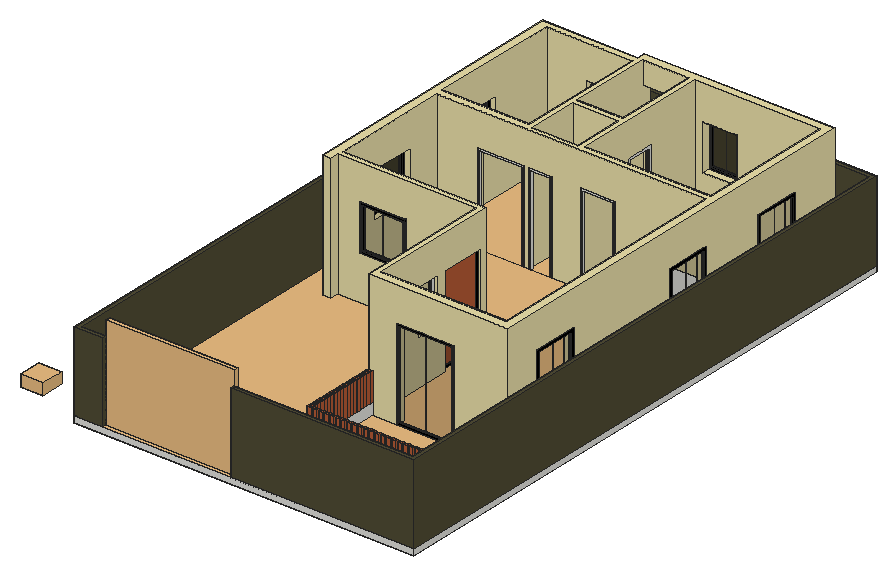
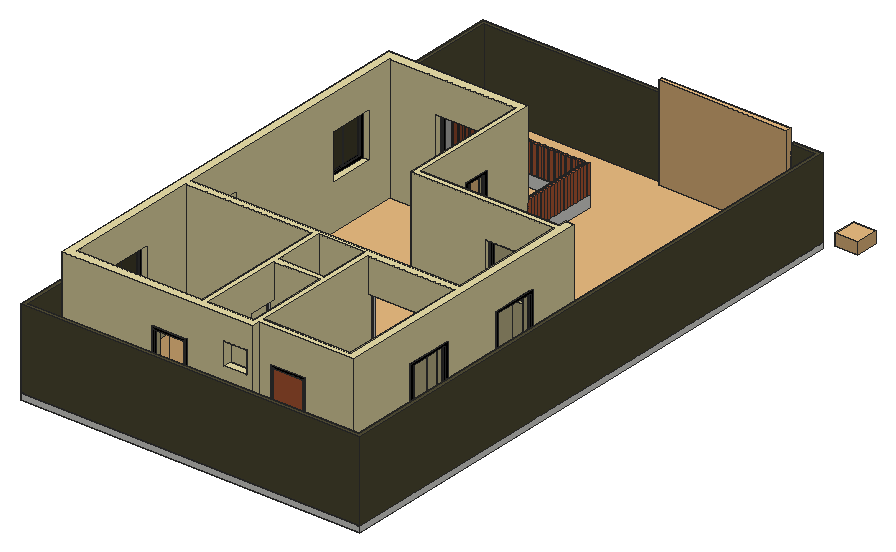
# SketchUp Ruby script. Lengths in inches.
U = 1.inch
M = Sketchup.active_model
def pt(a) = Geom::Point3d.new(a.map { |v| v * U })
def face(e, loops, mat)
  f = e.add_face(loops[0].map { |a| pt(a) })
  loops[1..].each { |l| e.add_face(l.map { |a| pt(a) }).erase! }
  f.material = f.back_material = mat if mat
  f
end
# faces: each face lists its corners as indices into pts; further lists are holes
def faces(e, pts, list, mat = nil) = list.each { |f| face(e, (f[0].is_a?(Array) ? f : [f]).map { |l| l.map { |i| pts[i] } }, mat) }
# xy, xz, yz: faces in a plane at the given z, y or x. An outline is a flat list of corners, or four numbers for a rectangle; further outlines are holes
def ring(l) = l.size == 4 ? [[l[0], l[1]], [l[2], l[1]], [l[2], l[3]], [l[0], l[3]]] : l.each_slice(2).to_a
def flat(e, list, mat, &to3) = list.each { |f| face(e, (f[0].is_a?(Array) ? f : [f]).map { |l| ring(l).map { |u, v| to3.(u, v) } }, mat) }
def xy(e, z, list, mat = nil) = flat(e, list, mat) { |x, y| [x, y, z] }
def xz(e, y, list, mat = nil) = flat(e, list, mat) { |x, z| [x, y, z] }
def yz(e, x, list, mat = nil) = flat(e, list, mat) { |y, z| [x, y, z] }
def lines(e, pts, list) = list.each { |a, b| e.add_line(pt(pts[a]), pt(pts[b])) }
# prism: a flat outline (further loops are holes) pulled along v
def prism(e, loops, v, mat = nil)
  f = face(e, loops, mat); d = Geom::Vector3d.new(v.map { |x| x * U })
  f.pushpull(f.normal.samedirection?(d) ? d.length : -d.length)
end
def box(e, o, s, mat = nil) = prism(e, [[o, [o[0] + s[0], o[1], o[2]], [o[0] + s[0], o[1] + s[1], o[2]], [o[0], o[1] + s[1], o[2]]]], [0, 0, s[2]], mat)
def at(x, y, z, deg = 0) = Geom::Transformation.translation(pt([x, y, z])) * Geom::Transformation.rotation(ORIGIN, Z_AXIS, deg.degrees)
def axes(o, x, y, z) = Geom::Transformation.new([*x, 0, *y, 0, *z, 0, *pt(o).to_a, 1])
def part(name) = M.definitions.add(name)
# library, detail: a bought-in or finely detailed component or shape, given as its bounding box
def library(name, o, s) = part(name).tap { |d| box(d.entities, o, s) }
def detail(e, o, s) = box(e.add_group.entities, o, s)
def put(e, d, t, mat = nil) = e.add_instance(d, t).tap { |i| i.material = mat if mat }
def group(e, t, mat = nil) = e.add_group.tap { |g| g.transformation = t; g.material = mat if mat }.entities
root = M.entities
M.materials.add("METAL").color = [0, 0, 0]
M.materials.add("WALL PAINT").color = [235, 224, 170]
M.materials.add("WALL PAINT\#1").color = [80, 76, 53]
M.materials.add("WHITE FLOOR").color = [250, 250, 243]
M.materials.add("glass").color = [0, 0, 0]
M.materials["glass"].alpha = 0.1
M.materials.add("wood").color = [181, 91, 54]
c1 = part("Group\#111")
box(c1.entities,[0,0,0],[4.5,2.78,30])
c2 = part("Stair tread")
box(c2.entities,[0,0,0],[12,39.4375,7])
c3 = library("gate 119k",[0,1.18,0],[135.43,4.73,99.21])
c4 = library("Group\#1",[0,0,0],[357,609,0.01])
c5 = library("Dome Light",[-12,-12,0],[24,24,12])
c6 = part("Component\#2")
box(c6.entities,[0,0,0],[36,36,19.4375])
prism(root,[[[164.87,4.5,0],[352.5,4.5,0],[352.5,604.5,0],[4.5,604.5,0],[4.5,4.5,0],[29.875,4.5,0],[29.875,0,0],[0,0,0],[0,609,0],[357,609,0],[357,0,0],[164.87,0,0]]],[0,0,84],"WALL PAINT\#1")
g1 = group(root,at(32,74,-6))
xy(g1,0,[[-32,-74,325,535]])
xy(g1,6,[[-32,-74,325,535]],"WHITE FLOOR")
xz(g1,-74,[[-32,0,325,6]])
xz(g1,535,[[-32,0,325,6]])
yz(g1,-32,[[-74,0,535,6]])
yz(g1,325,[[-74,0,535,6]])
g2 = group(root,at(216,154.5,0))
prism(g2,[[[60,0,95.4375],[0,0,95.4375],[0,0,0],[60,0,0]],[[58,0,2],[2,0,2],[2,0,93.4375],[58,0,93.4375]]],[0,2,0],"METAL")
g3 = group(root,at(138,426,0))
prism(g3,[[[2,2,0],[0,2,0],[0,2,95.4375],[24,2,95.4375],[24,2,0],[22,2,0],[22,2,93.4375],[2,2,93.4375]]],[0,-2,0])
p = [[2,0,0],[22,0,0]]
lines(g3,p,[[0,1]])
g4 = group(root,at(192,426,0))
prism(g4,[[[2,2,0],[0,2,0],[0,2,95.4375],[36,2,95.4375],[36,2,0],[34,2,0],[34,2,93.4375],[2,2,93.4375]]],[0,-2,0])
p = [[2,0,0],[34,0,0]]
lines(g4,p,[[0,1]])
g5 = group(root,at(186,74,0))
xy(g5,0,[[0,0,0,80.5,4.5,80.5,4.5,4.5,142.5,4.5,142.5,80.5,147,80.5,147,0]])
xy(g5,12,[[0,0,147,0,147,4.5,4.5,4.5,4.5,77.72,0,77.72]])
xy(g5,48,[[142.5,4.5,147,80.5]])
xz(g5,0,[[0,0,147,12]])
xz(g5,4.5,[[4.5,0,142.5,12],[142.5,12,147,48]])
xz(g5,80.5,[[0,0,4.5,12],[142.5,0,147,48]])
yz(g5,0,[[0,0,80.5,12]])
yz(g5,4.5,[[4.5,0,80.5,12]])
yz(g5,142.5,[[4.5,0,80.5,48]])
yz(g5,147,[[0,0,80.5,0,80.5,48,4.5,48,4.5,12,0,12]])
put(g5,c1,at(0,77.72,12),"wood")
put(g5,c1,at(0,73.4,12),"wood")
put(g5,c1,at(0,69.08,12),"wood")
g6 = group(g5,at(0,64.77,12),"wood")
box(g6,[0,0,0],[4.5,2.78,30])
put(g5,c1,at(0,60.45,12),"wood")
put(g5,c1,at(0,56.13,12),"wood")
put(g5,c1,at(0,51.8125,12),"wood")
put(g5,c1,at(0,47.49,12),"wood")
put(g5,c1,at(0,43.18,12),"wood")
put(g5,c1,at(0,38.86,12),"wood")
put(g5,c1,at(0,34.54,12),"wood")
put(g5,c1,at(0,30.22,12),"wood")
put(g5,c1,at(0,25.91,12),"wood")
put(g5,c1,at(0,21.59,12),"wood")
put(g5,c1,at(0,17.27,12),"wood")
put(g5,c1,at(0,12.95,12),"wood")
put(g5,c1,at(0,8.64,12),"wood")
put(g5,c1,at(0,4.32,12),"wood")
put(g5,c1,at(0,0,12),"wood")
put(g5,c1,at(5.9375,0,12),"wood")
put(g5,c1,at(11.875,0,12),"wood")
put(g5,c1,at(17.8125,0,12),"wood")
put(g5,c1,at(23.75,0,12),"wood")
put(g5,c1,at(29.6875,0,12),"wood")
put(g5,c1,at(35.625,0,12),"wood")
put(g5,c1,at(41.5625,0,12),"wood")
put(g5,c1,at(47.5,0,12),"wood")
put(g5,c1,at(53.4375,0,12),"wood")
put(g5,c1,at(59.375,0,12),"wood")
put(g5,c1,at(65.3125,0,12),"wood")
put(g5,c1,at(71.25,0,12),"wood")
put(g5,c1,at(77.1875,0,12),"wood")
put(g5,c1,at(83.125,0,12),"wood")
put(g5,c1,at(89.0625,0,12),"wood")
put(g5,c1,at(95,0,12),"wood")
put(g5,c1,at(100.9375,0,12),"wood")
put(g5,c1,at(106.875,0,12),"wood")
put(g5,c1,at(112.8125,0,12),"wood")
put(g5,c1,at(118.75,0,12),"wood")
put(g5,c1,at(124.6875,0,12),"wood")
put(g5,c1,at(130.625,0,12),"wood")
put(g5,c1,at(136.5625,0,12),"wood")
put(g5,c1,at(142.5,0,12),"wood")
put(root,c2,at(228,390,0))
put(root,c3,at(29.875,3.32,0))
g7 = group(root,at(32,154.5,0))
xy(g7,0,[[244,0,244,9,292,9,292,271.5,196,271.5,196,277.5,292,277.5,292,421.5,160,421.5,160,364.5,154,364.5,154,421.5,106,421.5,106,271.5,100,271.5,100,430.5,301,430.5,301,0],[154,0,154,92.9375,160,92.9375,160,9,184,9,184,0],[0,132,0,421.5,52,421.5,52,415.5,9,415.5,9,278.5,52,278.5,52,271.5,9,271.5,9,147,160,147,160,141,9,141,9,132]],"WALL PAINT")
xy(g7,47.4375,[[292,36.07,301,84.07],[154,57,160,83.9375],[33,141,81,147],[0,188.67,9,236.67],[292,210.97,301,258.97],
  [0,301.21,9,349.21],[292,327.45,301,375.45],[169,421.5,205,430.5]],"WALL PAINT")
xy(g7,83.4375,[[106,421.5,130,430.5]],"WALL PAINT")
xy(g7,95.4375,[[184,0,244,9],[292,36.07,301,84.07],[154,57,160,83.9375],[154,92.9375,160,141],[33,141,81,147],
  [0,188.67,9,236.67],[292,210.97,301,258.97],[52,271.5,100,278.5],[106,271.5,130,275.5],[160,271.5,196,277.5],
  [0,301.21,9,349.21],[292,327.45,301,375.45],[154,334.5,160,364.5],[52,415.5,88,421.5],[169,421.5,205,430.5]],"WALL PAINT")
xy(g7,107.4375,[[106,421.5,130,430.5]],"WALL PAINT")
xy(g7,131.4375,[[[154,0,301,0,301,430.5,100,430.5,100,421.5,0,421.5,0,132,9,132,9,141,154,141],[160,9,160,147,9,147,9,271.5,292,271.5,292,9],[160,277.5,292,421.5],[9,278.5,100,415.5],[106,334.5,154,421.5],[106,275.5,154,328.5]]],"WALL PAINT")
xz(g7,0,[[154,0,184,0,184,95.4375,244,95.4375,244,0,301,0,301,131.4375,154,131.4375]],"WALL PAINT")
xz(g7,9,[[160,0,160,131.4375,292,131.4375,292,0,244,0,244,95.4375,184,95.4375,184,0]],"WALL PAINT")
xz(g7,36.07,[[292,47.4375,301,95.4375]],"WALL PAINT")
xz(g7,57,[[154,47.4375,160,95.4375]],"WALL PAINT")
xz(g7,83.9375,[[154,47.4375,160,95.4375]],"WALL PAINT")
xz(g7,84.07,[[292,47.4375,301,95.4375]],"WALL PAINT")
xz(g7,92.9375,[[154,0,160,95.4375]],"WALL PAINT")
xz(g7,132,[[0,0,9,131.4375]],"WALL PAINT")
xz(g7,141,[[[9,0,160,0,160,95.4375,154,95.4375,154,131.4375,9,131.4375],[33,47.4375,81,95.4375]]],"WALL PAINT")
xz(g7,147,[[[9,0,160,131.4375],[33,47.4375,81,95.4375]]],"WALL PAINT")
xz(g7,188.67,[[0,47.4375,9,95.4375]],"WALL PAINT")
xz(g7,210.97,[[292,47.4375,301,95.4375]],"WALL PAINT")
xz(g7,236.67,[[0,47.4375,9,95.4375]],"WALL PAINT")
xz(g7,258.97,[[292,47.4375,301,95.4375]],"WALL PAINT")
xz(g7,271.5,[[9,0,52,0,52,95.4375,100,95.4375,100,0,106,0,106,95.4375,130,95.4375,130,0,160,0,160,95.4375,196,95.4375,196,0,292,0,292,131.4375,9,131.4375]],"WALL PAINT")
xz(g7,275.5,[[130,0,130,95.4375,106,95.4375,106,131.4375,154,131.4375,154,0]],"WALL PAINT")
xz(g7,277.5,[[196,0,196,95.4375,160,95.4375,160,131.4375,292,131.4375,292,0]],"WALL PAINT")
xz(g7,278.5,[[9,0,9,131.4375,100,131.4375,100,95.4375,52,95.4375,52,0]],"WALL PAINT")
xz(g7,301.21,[[0,47.4375,9,95.4375]],"WALL PAINT")
xz(g7,327.45,[[292,47.4375,301,95.4375]],"WALL PAINT")
xz(g7,328.5,[[106,0,154,131.4375]],"WALL PAINT")
xz(g7,334.5,[[106,0,106,131.4375,154,131.4375,154,95.4375,160,95.4375,160,0]],"WALL PAINT")
xz(g7,349.21,[[0,47.4375,9,95.4375]],"WALL PAINT")
xz(g7,364.5,[[154,0,160,95.4375]],"WALL PAINT")
xz(g7,375.45,[[292,47.4375,301,95.4375]],"WALL PAINT")
xz(g7,415.5,[[9,0,52,0,52,95.4375,88,95.4375,88,0,100,0,100,131.4375,9,131.4375]],"WALL PAINT")
xz(g7,421.5,[[0,0,0,131.4375,100,131.4375,100,0,88,0,88,95.4375,52,95.4375,52,0],[106,0,154,0,154,131.4375,106,131.4375,106,107.4375,130,107.4375,130,83.4375,106,83.4375],[[160,0,292,131.4375],[169,47.4375,205,95.4375]]],"WALL PAINT")
xz(g7,430.5,[[[100,0,301,131.4375],[169,47.4375,205,95.4375],[106,83.4375,130,107.4375]]],"WALL PAINT")
yz(g7,0,[[[132,0,421.5,131.4375],[301.21,47.4375,349.21,95.4375],[188.67,47.4375,236.67,95.4375]]],"WALL PAINT")
yz(g7,9,[[132,0,141,131.4375],[[147,0,271.5,131.4375],[188.67,47.4375,236.67,95.4375]],[[278.5,0,415.5,131.4375],[301.21,47.4375,349.21,95.4375]]],"WALL PAINT")
yz(g7,33,[[141,47.4375,147,95.4375]],"WALL PAINT")
yz(g7,52,[[271.5,0,278.5,95.4375],[415.5,0,421.5,95.4375]],"WALL PAINT")
yz(g7,81,[[141,47.4375,147,95.4375]],"WALL PAINT")
yz(g7,88,[[415.5,0,421.5,95.4375]],"WALL PAINT")
yz(g7,100,[[271.5,0,271.5,95.4375,278.5,95.4375,278.5,131.4375,415.5,131.4375,415.5,0],[421.5,0,430.5,131.4375]],"WALL PAINT")
yz(g7,106,[[271.5,0,328.5,0,328.5,131.4375,275.5,131.4375,275.5,95.4375,271.5,95.4375],[334.5,0,421.5,0,421.5,83.4375,430.5,83.4375,430.5,107.4375,421.5,107.4375,421.5,131.4375,334.5,131.4375]],"WALL PAINT")
yz(g7,130,[[271.5,0,275.5,95.4375],[421.5,83.4375,430.5,107.4375]],"WALL PAINT")
yz(g7,154,[[[0,0,0,131.4375,141,131.4375,141,95.4375,92.9375,95.4375,92.9375,0],[57,47.4375,83.9375,95.4375]],[275.5,0,328.5,131.4375],[364.5,0,364.5,95.4375,334.5,95.4375,334.5,131.4375,421.5,131.4375,421.5,0]],"WALL PAINT")
yz(g7,160,[[[9,0,92.9375,0,92.9375,95.4375,141,95.4375,141,0,147,0,147,131.4375,9,131.4375],[57,47.4375,83.9375,95.4375]],[271.5,0,334.5,0,334.5,95.4375,364.5,95.4375,364.5,0,421.5,0,421.5,131.4375,277.5,131.4375,277.5,95.4375,271.5,95.4375]],"WALL PAINT")
yz(g7,169,[[421.5,47.4375,430.5,95.4375]],"WALL PAINT")
yz(g7,184,[[0,0,9,95.4375]],"WALL PAINT")
yz(g7,196,[[271.5,0,277.5,95.4375]],"WALL PAINT")
yz(g7,205,[[421.5,47.4375,430.5,95.4375]],"WALL PAINT")
yz(g7,244,[[0,0,9,95.4375]],"WALL PAINT")
yz(g7,292,[[[9,0,271.5,131.4375],[36.07,47.4375,84.07,95.4375],[210.97,47.4375,258.97,95.4375]],[[277.5,0,421.5,131.4375],[327.45,47.4375,375.45,95.4375]]],"WALL PAINT")
yz(g7,301,[[[0,0,430.5,131.4375],[36.07,47.4375,84.07,95.4375],[210.97,47.4375,258.97,95.4375],[327.45,47.4375,375.45,95.4375]]],"WALL PAINT")
p = [[244,0,0],[184,0,0]]
lines(g7,p,[[0,1]])
put(root,c4,at(0,0,0))
g8 = group(root,at(84,576,0))
xy(g8,0,[[0,-2,36,0]])
xy(g8,2,[[2,-2,34,0]])
xy(g8,93.4375,[[2,-2,34,0]])
xy(g8,95.4375,[[0,-2,36,0]])
xz(g8,-2,[[[0,0,36,95.4375],[2,2,34,93.4375]]])
xz(g8,0,[[[0,0,36,95.4375],[2,2,34,93.4375]]],"METAL")
yz(g8,0,[[-2,0,0,95.4375]])
yz(g8,2,[[-2,2,0,93.4375]])
yz(g8,34,[[-2,2,0,93.4375]])
yz(g8,36,[[-2,0,0,95.4375]])
g9 = group(root,at(186,247.4375,0))
prism(g9,[[[0,48.0625,95.4375],[0,48.0625,0],[0,0,0],[0,0,95.4375]],[[0,46.0625,93.4375],[0,2,93.4375],[0,2,2],[0,46.0625,2]]],[2,0,0],"METAL")
g10 = group(root,at(84,426,0))
prism(g10,[[[0,0,0],[2,0,0],[2,0,93.4375],[46,0,93.4375],[46,0,0],[48,0,0],[48,0,95.4375],[0,0,95.4375]]],[0,2,0])
p = [[2,0,0],[46,0,0]]
lines(g10,p,[[0,1]])
g11 = group(root,at(192,489,0))
prism(g11,[[[0,0,0],[0,30,0],[0,30,95.4375],[0,0,95.4375]],[[0,28,93.4375],[0,28,2],[0,2,2],[0,2,93.4375]]],[-2,0,0])
g12 = group(root,at(218,155.875,2))
box(g12,[0,0,0],[28,0.31,91.4375],"glass")
g13 = group(root,at(246,155.56,2))
box(g13,[0,0,0],[28,0.31,91.4375],"glass")
g14 = group(root,at(186,249.4375,2),"wood")
box(g14,[0,0,0],[0.71,44.0625,91.4375])
g15 = group(root,at(86,576,2),"wood")
box(g15,[0,-0.71,0],[32,0.71,91.4375])
put(root,c2,at(240,390,7))
put(root,c5,at(-38.72,4.5,13.38))
put(root,c2,at(252,390,14))
put(root,c2,at(264,390,21))
put(root,c2,at(276,390,28))
put(root,c6,at(288,390,35))
g16 = group(root,at(186,285.01,45.95),"METAL")
box(g16,[-0.625,0,0],[0.625,1.375,6])
g17 = group(root,at(31.22,343.17,47.4375))
prism(g17,[[[-1,48,0],[-1,0,0],[-1,0,48],[-1,48,48]],[[-1,2,46],[-1,2,2],[-1,46,2],[-1,46,46]]],[3.78,0,0],"METAL")
g18 = group(root,at(31.22,455.71,47.4375))
prism(g18,[[[-1,48,0],[-1,0,0],[-1,0,48],[-1,48,48]],[[-1,2,46],[-1,2,2],[-1,46,2],[-1,46,46]]],[3.78,0,0],"METAL")
g19 = group(root,at(201,585.625,47.4375))
prism(g19,[[[36,-2,0],[36,-2,48],[0,-2,48],[0,-2,0]],[[2,-2,2],[2,-2,46],[34,-2,46],[34,-2,2]]],[0,3,0],"METAL")
g20 = group(root,at(65,295.5,47.4375))
prism(g20,[[[0,1.5,48],[48,1.5,48],[48,1.5,0],[0,1.5,0]],[[46,1.5,46],[2,1.5,46],[2,1.5,2],[46,1.5,2]]],[0,-3,0],"METAL")
g21 = group(root,at(186,211.5,47.4375))
xy(g21,0,[[-1.5,0,1.5,26.9375]])
xy(g21,2,[[-1.5,2,1.5,24.9375]])
xy(g21,46,[[-1.5,2,1.5,24.9375]])
xy(g21,48,[[-1.5,0,1.5,26.9375]])
xz(g21,0,[[-1.5,0,1.5,48]])
xz(g21,2,[[-1.5,2,1.5,46]])
xz(g21,24.9375,[[-1.5,2,1.5,46]])
xz(g21,26.9375,[[-1.5,0,1.5,48]])
yz(g21,-1.5,[[[0,0,26.9375,48],[2,2,24.9375,46]]],"METAL")
yz(g21,1.5,[[[0,0,26.9375,48],[2,2,24.9375,46]]])
g22 = group(root,at(333,190.57,47.4375))
prism(g22,[[[-1.5,0,0],[-1.5,0,48],[-1.5,48,48],[-1.5,48,0]],[[-1.5,46,2],[-1.5,46,46],[-1.5,2,46],[-1.5,2,2]]],[3,0,0],"METAL")
g23 = group(root,at(333,365.47,47.4375))
prism(g23,[[[-1.5,48,0],[-1.5,0,0],[-1.5,0,48],[-1.5,48,48]],[[-1.5,46,2],[-1.5,46,46],[-1.5,2,46],[-1.5,2,2]]],[3,0,0],"METAL")
g24 = group(root,at(333,481.95,47.4375))
prism(g24,[[[-1.5,0,0],[-1.5,0,48],[-1.5,48,48],[-1.5,48,0]],[[-1.5,46,46],[-1.5,2,46],[-1.5,2,2],[-1.5,46,2]]],[3,0,0],"METAL")
g25 = group(root,at(32.47,479.71,49.4375))
box(g25,[-0.31,0,0],[0.31,22,44],"glass")
g26 = group(root,at(32.16,457.71,49.4375))
box(g26,[-0.31,0,0],[0.31,22,44],"glass")
g27 = group(root,at(32.28,367.17,49.4375))
box(g27,[0,0,0],[0.31,22,44],"glass")
g28 = group(root,at(31.97,345.17,49.4375))
box(g28,[0,0,0],[0.31,22,44],"glass")
g29 = group(root,at(67,295.4375,49.4375))
box(g29,[0,0,0],[22,0.31,44],"glass")
g30 = group(root,at(89,295.12,49.4375))
box(g30,[0,0,0],[22,0.31,44],"glass")
g31 = group(root,at(185.9375,213.5,49.4375))
box(g31,[0,0,0],[0.31,22.9375,44],"glass")
g32 = group(root,at(332.8125,192.57,49.4375))
box(g32,[-0.31,0,0],[0.31,22,44],"glass")
g33 = group(root,at(333.13,214.57,49.4375))
box(g33,[-0.31,0,0],[0.31,22,44],"glass")
g34 = group(root,at(332.75,367.47,49.4375))
box(g34,[-0.31,0,0],[0.31,22,44],"glass")
g35 = group(root,at(333.06,389.47,49.4375))
box(g35,[-0.31,0,0],[0.31,22,44],"glass")
g36 = group(root,at(332.75,483.95,49.4375))
box(g36,[-0.31,0,0],[0.31,22,44],"glass")
g37 = group(root,at(333.06,505.95,49.4375))
box(g37,[-0.31,0,0],[0.31,22,44],"glass")
g38 = group(root,at(219,585.0625,49.4375))
box(g38,[0,-0.31,0],[16,0.31,44],"glass")
g39 = group(root,at(203,585.38,49.4375))
box(g39,[0,-0.31,0],[16,0.31,44],"glass")
